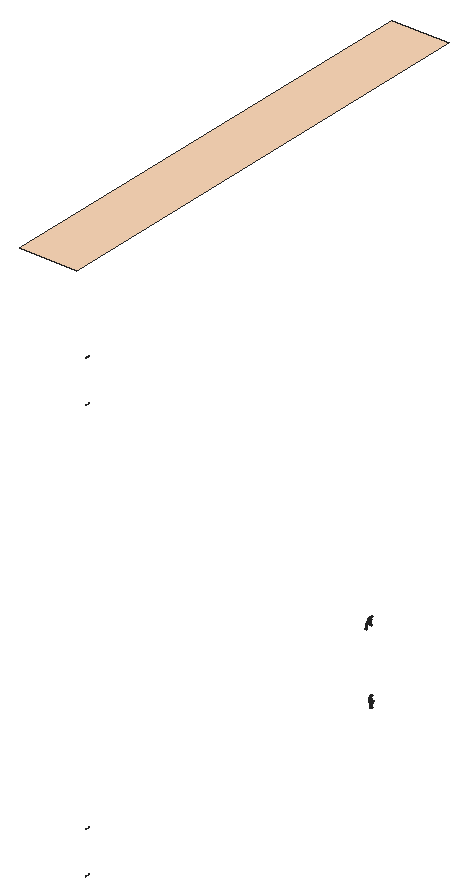
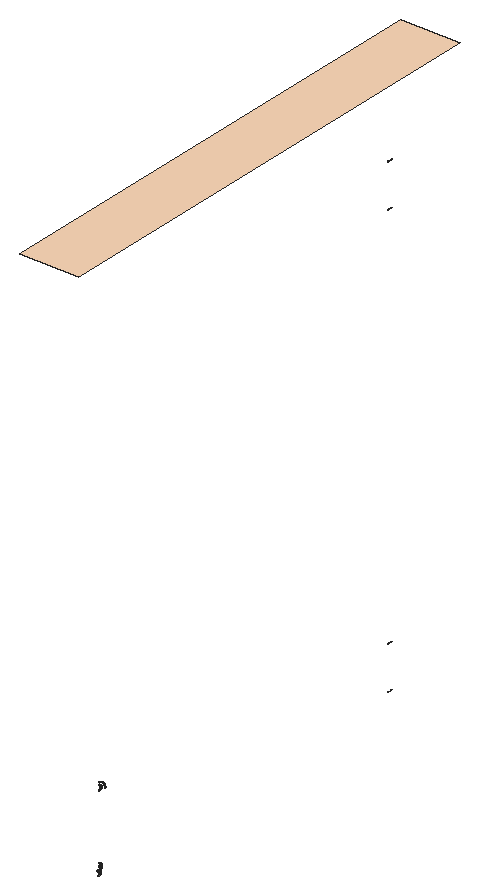
# SketchUp Ruby script. Lengths in inches.
U = 1.inch
M = Sketchup.active_model
def pt(a) = Geom::Point3d.new(a.map { |v| v * U })
def face(e, loops, mat)
  f = e.add_face(loops[0].map { |a| pt(a) })
  loops[1..].each { |l| e.add_face(l.map { |a| pt(a) }).erase! }
  f.material = f.back_material = mat if mat
  f
end
# faces: each face lists its corners as indices into pts; further lists are holes
def faces(e, pts, list, mat = nil) = list.each { |f| face(e, (f[0].is_a?(Array) ? f : [f]).map { |l| l.map { |i| pts[i] } }, mat) }
# xy, xz, yz: faces in a plane at the given z, y or x. An outline is a flat list of corners, or four numbers for a rectangle; further outlines are holes
def ring(l) = l.size == 4 ? [[l[0], l[1]], [l[2], l[1]], [l[2], l[3]], [l[0], l[3]]] : l.each_slice(2).to_a
def flat(e, list, mat, &to3) = list.each { |f| face(e, (f[0].is_a?(Array) ? f : [f]).map { |l| ring(l).map { |u, v| to3.(u, v) } }, mat) }
def xy(e, z, list, mat = nil) = flat(e, list, mat) { |x, y| [x, y, z] }
def xz(e, y, list, mat = nil) = flat(e, list, mat) { |x, z| [x, y, z] }
def yz(e, x, list, mat = nil) = flat(e, list, mat) { |y, z| [x, y, z] }
def lines(e, pts, list) = list.each { |a, b| e.add_line(pt(pts[a]), pt(pts[b])) }
# prism: a flat outline (further loops are holes) pulled along v
def prism(e, loops, v, mat = nil)
  f = face(e, loops, mat); d = Geom::Vector3d.new(v.map { |x| x * U })
  f.pushpull(f.normal.samedirection?(d) ? d.length : -d.length)
end
def box(e, o, s, mat = nil) = prism(e, [[o, [o[0] + s[0], o[1], o[2]], [o[0] + s[0], o[1] + s[1], o[2]], [o[0], o[1] + s[1], o[2]]]], [0, 0, s[2]], mat)
def at(x, y, z, deg = 0) = Geom::Transformation.translation(pt([x, y, z])) * Geom::Transformation.rotation(ORIGIN, Z_AXIS, deg.degrees)
def axes(o, x, y, z) = Geom::Transformation.new([*x, 0, *y, 0, *z, 0, *pt(o).to_a, 1])
def part(name) = M.definitions.add(name)
# library, detail: a bought-in or finely detailed component or shape, given as its bounding box
def library(name, o, s) = part(name).tap { |d| box(d.entities, o, s) }
def detail(e, o, s) = box(e.add_group.entities, o, s)
def put(e, d, t, mat = nil) = e.add_instance(d, t).tap { |i| i.material = mat if mat }
def group(e, t, mat = nil) = e.add_group.tap { |g| g.transformation = t; g.material = mat if mat }.entities
root = M.entities
M.materials.add("Material \#1").color = [140, 140, 140]
M.materials.add("[0027_PeachPuff]").color = [255, 218, 185]
xy(root,47.1053,[[362.6071,164.2401,362.6036,164.2537,362.604,164.275],[362.6071,164.2401,362.604,164.275,362.6071,164.2627],[362.6071,164.2401,362.6071,164.2627,362.6107,164.2537],[362.6036,164.2537,362.6005,164.293,362.6012,164.3103],[362.6036,164.2537,362.6012,164.3103,362.604,164.275],
  [362.6107,164.2537,362.6071,164.2627,362.6103,164.275],[362.6107,164.2537,362.6103,164.275,362.6137,164.293],[362.6103,164.275,362.6131,164.3103,362.6137,164.293],[362.6005,164.293,362.5982,164.3532,362.5991,164.3645],[362.6005,164.293,362.5991,164.3645,362.6012,164.3103],
  [362.6137,164.293,362.6131,164.3103,362.616,164.3532],[362.6131,164.3103,362.6152,164.3645,362.616,164.3532],[362.5982,164.3532,362.597,164.427,362.598,164.431],[362.5982,164.3532,362.598,164.431,362.5991,164.3645],[362.616,164.3532,362.6152,164.3645,362.6173,164.427],
  [362.6152,164.3645,362.6163,164.431,362.6173,164.427],[362.597,164.427,362.597,164.5056,362.598,164.5017],[362.597,164.427,362.598,164.5017,362.598,164.431],[362.6173,164.427,362.6163,164.431,362.6173,164.5056],[362.6163,164.431,362.6163,164.5017,362.6173,164.5056],
  [362.598,164.5017,362.597,164.5056,362.5991,164.5681],[362.6163,164.5017,362.6152,164.5681,362.616,164.5795],[362.6163,164.5017,362.616,164.5795,362.6173,164.5056],[362.597,164.5056,362.5982,164.5795,362.5991,164.5681],[362.5991,164.5681,362.5982,164.5795,362.6012,164.6223],
  [362.6152,164.5681,362.6131,164.6223,362.6137,164.6396],[362.6152,164.5681,362.6137,164.6396,362.616,164.5795],[362.5982,164.5795,362.6005,164.6396,362.6012,164.6223],[362.6012,164.6223,362.6005,164.6396,362.604,164.6577],[362.6131,164.6223,362.6103,164.6577,362.6107,164.6789],
  [362.6131,164.6223,362.6107,164.6789,362.6137,164.6396],[362.6005,164.6396,362.6036,164.6789,362.604,164.6577],[362.604,164.6577,362.6036,164.6789,362.6071,164.6699],[362.6103,164.6577,362.6071,164.6699,362.6071,164.6926],[362.6103,164.6577,362.6071,164.6926,362.6107,164.6789],
  [362.6071,164.6699,362.6036,164.6789,362.6071,164.6926]],"Material \#1")
xy(root,47.125,[[362.6071,164.2401,362.6071,164.2627,362.6036,164.2537],[362.6071,164.2401,362.6103,164.275,362.6071,164.2627],[362.6071,164.2401,362.6107,164.2537,362.6103,164.275],[362.6036,164.2537,362.604,164.275,362.6005,164.293],[362.6036,164.2537,362.6071,164.2627,362.604,164.275],
  [362.6107,164.2537,362.6131,164.3103,362.6103,164.275],[362.6107,164.2537,362.6137,164.293,362.6131,164.3103],[362.604,164.275,362.6012,164.3103,362.6005,164.293],[362.6005,164.293,362.6012,164.3103,362.5982,164.3532],[362.6137,164.293,362.6152,164.3645,362.6131,164.3103],
  [362.6137,164.293,362.616,164.3532,362.6152,164.3645],[362.6012,164.3103,362.5991,164.3645,362.5982,164.3532],[362.5982,164.3532,362.5991,164.3645,362.597,164.427],[362.616,164.3532,362.6163,164.431,362.6152,164.3645],[362.616,164.3532,362.6173,164.427,362.6163,164.431],
  [362.5991,164.3645,362.598,164.431,362.597,164.427],[362.597,164.427,362.598,164.431,362.597,164.5056],[362.6173,164.427,362.6163,164.5017,362.6163,164.431],[362.6173,164.427,362.6173,164.5056,362.6163,164.5017],[362.598,164.431,362.598,164.5017,362.597,164.5056],
  [362.598,164.5017,362.5982,164.5795,362.597,164.5056],[362.598,164.5017,362.5991,164.5681,362.5982,164.5795],[362.6163,164.5017,362.6173,164.5056,362.6152,164.5681],[362.6173,164.5056,362.616,164.5795,362.6152,164.5681],[362.5991,164.5681,362.6005,164.6396,362.5982,164.5795],
  [362.5991,164.5681,362.6012,164.6223,362.6005,164.6396],[362.6152,164.5681,362.616,164.5795,362.6131,164.6223],[362.616,164.5795,362.6137,164.6396,362.6131,164.6223],[362.6012,164.6223,362.6036,164.6789,362.6005,164.6396],[362.6012,164.6223,362.604,164.6577,362.6036,164.6789],
  [362.6131,164.6223,362.6137,164.6396,362.6103,164.6577],[362.6137,164.6396,362.6107,164.6789,362.6103,164.6577],[362.604,164.6577,362.6071,164.6926,362.6036,164.6789],[362.604,164.6577,362.6071,164.6699,362.6071,164.6926],[362.6103,164.6577,362.6107,164.6789,362.6071,164.6699],
  [362.6071,164.6699,362.6107,164.6789,362.6071,164.6926]],"Material \#1")
xy(root,51.5484,[[362.6071,164.2401,362.6036,164.2537,362.6071,164.2627],[362.6071,164.2401,362.6071,164.2627,362.6103,164.275],[362.6071,164.2401,362.6103,164.275,362.6107,164.2537],[362.6036,164.2537,362.6005,164.293,362.604,164.275],[362.6036,164.2537,362.604,164.275,362.6071,164.2627],
  [362.6107,164.2537,362.6103,164.275,362.6131,164.3103],[362.6107,164.2537,362.6131,164.3103,362.6137,164.293],[362.604,164.275,362.6005,164.293,362.6012,164.3103],[362.6005,164.293,362.5982,164.3532,362.6012,164.3103],[362.6137,164.293,362.6131,164.3103,362.6152,164.3645],
  [362.6137,164.293,362.6152,164.3645,362.616,164.3532],[362.6012,164.3103,362.5982,164.3532,362.5991,164.3645],[362.5982,164.3532,362.597,164.427,362.5991,164.3645],[362.616,164.3532,362.6152,164.3645,362.6163,164.431],[362.616,164.3532,362.6163,164.431,362.6173,164.427],
  [362.5991,164.3645,362.597,164.427,362.598,164.431],[362.597,164.427,362.597,164.5056,362.598,164.431],[362.6173,164.427,362.6163,164.431,362.6163,164.5017],[362.6173,164.427,362.6163,164.5017,362.6173,164.5056],[362.598,164.431,362.597,164.5056,362.598,164.5017],
  [362.598,164.5017,362.597,164.5056,362.5982,164.5794],[362.598,164.5017,362.5982,164.5794,362.5991,164.5681],[362.6163,164.5017,362.6152,164.5681,362.6173,164.5056],[362.6173,164.5056,362.6152,164.5681,362.616,164.5794],[362.5991,164.5681,362.5982,164.5794,362.6005,164.6396],
  [362.5991,164.5681,362.6005,164.6396,362.6012,164.6223],[362.6152,164.5681,362.6131,164.6223,362.616,164.5794],[362.616,164.5794,362.6131,164.6223,362.6137,164.6396],[362.6012,164.6223,362.6005,164.6396,362.6036,164.6789],[362.6012,164.6223,362.6036,164.6789,362.604,164.6577],
  [362.6131,164.6223,362.6103,164.6577,362.6137,164.6396],[362.6137,164.6396,362.6103,164.6577,362.6107,164.6789],[362.604,164.6577,362.6036,164.6789,362.6071,164.6926],[362.604,164.6577,362.6071,164.6926,362.6071,164.6699],[362.6103,164.6577,362.6071,164.6699,362.6107,164.6789],
  [362.6071,164.6699,362.6071,164.6926,362.6107,164.6789]],"Material \#1")
xy(root,51.5681,[[362.6071,164.2401,362.604,164.275,362.6036,164.2537],[362.6071,164.2401,362.6071,164.2627,362.604,164.275],[362.6071,164.2401,362.6107,164.2537,362.6071,164.2627],[362.6036,164.2537,362.6012,164.3103,362.6005,164.293],[362.6036,164.2537,362.604,164.275,362.6012,164.3103],
  [362.6107,164.2537,362.6103,164.275,362.6071,164.2627],[362.6107,164.2537,362.6137,164.293,362.6103,164.275],[362.6103,164.275,362.6137,164.293,362.6131,164.3103],[362.6005,164.293,362.5991,164.3645,362.5982,164.3532],[362.6005,164.293,362.6012,164.3103,362.5991,164.3645],
  [362.6137,164.293,362.616,164.3532,362.6131,164.3103],[362.6131,164.3103,362.616,164.3532,362.6152,164.3645],[362.5982,164.3532,362.598,164.431,362.597,164.427],[362.5982,164.3532,362.5991,164.3645,362.598,164.431],[362.616,164.3532,362.6173,164.427,362.6152,164.3645],
  [362.6152,164.3645,362.6173,164.427,362.6163,164.431],[362.597,164.427,362.598,164.431,362.598,164.5017],[362.597,164.427,362.598,164.5017,362.597,164.5056],[362.6173,164.427,362.6173,164.5056,362.6163,164.431],[362.6163,164.431,362.6173,164.5056,362.6163,164.5017],
  [362.598,164.5017,362.5991,164.5681,362.597,164.5056],[362.6163,164.5017,362.616,164.5794,362.6152,164.5681],[362.6163,164.5017,362.6173,164.5056,362.616,164.5794],[362.597,164.5056,362.5991,164.5681,362.5982,164.5794],[362.5991,164.5681,362.6012,164.6223,362.5982,164.5794],
  [362.6152,164.5681,362.6137,164.6396,362.6131,164.6223],[362.6152,164.5681,362.616,164.5794,362.6137,164.6396],[362.5982,164.5794,362.6012,164.6223,362.6005,164.6396],[362.6012,164.6223,362.604,164.6577,362.6005,164.6396],[362.6131,164.6223,362.6107,164.6789,362.6103,164.6577],
  [362.6131,164.6223,362.6137,164.6396,362.6107,164.6789],[362.6005,164.6396,362.604,164.6577,362.6036,164.6789],[362.604,164.6577,362.6071,164.6699,362.6036,164.6789],[362.6103,164.6577,362.6071,164.6926,362.6071,164.6699],[362.6103,164.6577,362.6107,164.6789,362.6071,164.6926],
  [362.6071,164.6699,362.6071,164.6926,362.6036,164.6789]],"Material \#1")
xy(root,91.4868,[[362.6071,164.2401,362.6036,164.2537,362.604,164.275],[362.6071,164.2401,362.604,164.275,362.6071,164.2627],[362.6071,164.2401,362.6071,164.2627,362.6107,164.2537],[362.6036,164.2537,362.6005,164.293,362.6012,164.3103],[362.6036,164.2537,362.6012,164.3103,362.604,164.275],
  [362.6107,164.2537,362.6071,164.2627,362.6103,164.275],[362.6107,164.2537,362.6103,164.275,362.6137,164.293],[362.6103,164.275,362.6131,164.3103,362.6137,164.293],[362.6005,164.293,362.5982,164.3532,362.5991,164.3645],[362.6005,164.293,362.5991,164.3645,362.6012,164.3103],
  [362.6137,164.293,362.6131,164.3103,362.616,164.3532],[362.6131,164.3103,362.6152,164.3645,362.616,164.3532],[362.5982,164.3532,362.597,164.427,362.598,164.431],[362.5982,164.3532,362.598,164.431,362.5991,164.3645],[362.616,164.3532,362.6152,164.3645,362.6173,164.427],
  [362.6152,164.3645,362.6163,164.431,362.6173,164.427],[362.597,164.427,362.597,164.5056,362.598,164.5017],[362.597,164.427,362.598,164.5017,362.598,164.431],[362.6173,164.427,362.6163,164.431,362.6173,164.5056],[362.6163,164.431,362.6163,164.5017,362.6173,164.5056],
  [362.598,164.5017,362.597,164.5056,362.5991,164.5681],[362.6163,164.5017,362.6152,164.5681,362.616,164.5794],[362.6163,164.5017,362.616,164.5794,362.6173,164.5056],[362.597,164.5056,362.5982,164.5794,362.5991,164.5681],[362.5991,164.5681,362.5982,164.5794,362.6012,164.6223],
  [362.6152,164.5681,362.6131,164.6223,362.6137,164.6396],[362.6152,164.5681,362.6137,164.6396,362.616,164.5794],[362.5982,164.5794,362.6005,164.6396,362.6012,164.6223],[362.6012,164.6223,362.6005,164.6396,362.604,164.6577],[362.6131,164.6223,362.6103,164.6577,362.6107,164.6789],
  [362.6131,164.6223,362.6107,164.6789,362.6137,164.6396],[362.6005,164.6396,362.6036,164.6789,362.604,164.6577],[362.604,164.6577,362.6036,164.6789,362.6071,164.6699],[362.6103,164.6577,362.6071,164.6699,362.6071,164.6926],[362.6103,164.6577,362.6071,164.6926,362.6107,164.6789],
  [362.6071,164.6699,362.6036,164.6789,362.6071,164.6926]],"Material \#1")
xy(root,91.5065,[[362.6071,164.2401,362.6071,164.2627,362.6036,164.2537],[362.6071,164.2401,362.6103,164.275,362.6071,164.2627],[362.6071,164.2401,362.6107,164.2537,362.6103,164.275],[362.6036,164.2537,362.604,164.275,362.6005,164.293],[362.6036,164.2537,362.6071,164.2627,362.604,164.275],
  [362.6107,164.2537,362.6131,164.3103,362.6103,164.275],[362.6107,164.2537,362.6137,164.293,362.6131,164.3103],[362.604,164.275,362.6012,164.3103,362.6005,164.293],[362.6005,164.293,362.6012,164.3103,362.5982,164.3532],[362.6137,164.293,362.6152,164.3645,362.6131,164.3103],
  [362.6137,164.293,362.616,164.3532,362.6152,164.3645],[362.6012,164.3103,362.5991,164.3645,362.5982,164.3532],[362.5982,164.3532,362.5991,164.3645,362.597,164.427],[362.616,164.3532,362.6163,164.431,362.6152,164.3645],[362.616,164.3532,362.6173,164.427,362.6163,164.431],
  [362.5991,164.3645,362.598,164.431,362.597,164.427],[362.597,164.427,362.598,164.431,362.597,164.5056],[362.6173,164.427,362.6163,164.5017,362.6163,164.431],[362.6173,164.427,362.6173,164.5056,362.6163,164.5017],[362.598,164.431,362.598,164.5017,362.597,164.5056],
  [362.598,164.5017,362.5982,164.5794,362.597,164.5056],[362.598,164.5017,362.5991,164.5681,362.5982,164.5794],[362.6163,164.5017,362.6173,164.5056,362.6152,164.5681],[362.6173,164.5056,362.616,164.5794,362.6152,164.5681],[362.5991,164.5681,362.6005,164.6396,362.5982,164.5794],
  [362.5991,164.5681,362.6012,164.6223,362.6005,164.6396],[362.6152,164.5681,362.616,164.5794,362.6131,164.6223],[362.616,164.5794,362.6137,164.6396,362.6131,164.6223],[362.6012,164.6223,362.6036,164.6789,362.6005,164.6396],[362.6012,164.6223,362.604,164.6577,362.6036,164.6789],
  [362.6131,164.6223,362.6137,164.6396,362.6103,164.6577],[362.6137,164.6396,362.6107,164.6789,362.6103,164.6577],[362.604,164.6577,362.6071,164.6926,362.6036,164.6789],[362.604,164.6577,362.6071,164.6699,362.6071,164.6926],[362.6103,164.6577,362.6107,164.6789,362.6071,164.6699],
  [362.6071,164.6699,362.6107,164.6789,362.6071,164.6926]],"Material \#1")
xy(root,95.9299,[[362.6071,164.2401,362.6036,164.2537,362.6071,164.2627],[362.6071,164.2401,362.6071,164.2627,362.6103,164.275],[362.6071,164.2401,362.6103,164.275,362.6107,164.2537],[362.6036,164.2537,362.6005,164.293,362.604,164.275],[362.6036,164.2537,362.604,164.275,362.6071,164.2627],
  [362.6107,164.2537,362.6103,164.275,362.6131,164.3103],[362.6107,164.2537,362.6131,164.3103,362.6137,164.293],[362.604,164.275,362.6005,164.293,362.6012,164.3103],[362.6005,164.293,362.5982,164.3532,362.6012,164.3103],[362.6137,164.293,362.6131,164.3103,362.6152,164.3645],
  [362.6137,164.293,362.6152,164.3645,362.616,164.3532],[362.6012,164.3103,362.5982,164.3532,362.5991,164.3645],[362.5982,164.3532,362.597,164.427,362.5991,164.3645],[362.616,164.3532,362.6152,164.3645,362.6163,164.431],[362.616,164.3532,362.6163,164.431,362.6173,164.427],
  [362.5991,164.3645,362.597,164.427,362.598,164.431],[362.597,164.427,362.597,164.5056,362.598,164.431],[362.6173,164.427,362.6163,164.431,362.6163,164.5017],[362.6173,164.427,362.6163,164.5017,362.6173,164.5056],[362.598,164.431,362.597,164.5056,362.598,164.5017],
  [362.598,164.5017,362.597,164.5056,362.5982,164.5794],[362.598,164.5017,362.5982,164.5794,362.5991,164.5681],[362.6163,164.5017,362.6152,164.5681,362.6173,164.5056],[362.6173,164.5056,362.6152,164.5681,362.616,164.5794],[362.5991,164.5681,362.5982,164.5794,362.6005,164.6396],
  [362.5991,164.5681,362.6005,164.6396,362.6012,164.6223],[362.6152,164.5681,362.6131,164.6223,362.616,164.5794],[362.616,164.5794,362.6131,164.6223,362.6137,164.6396],[362.6012,164.6223,362.6005,164.6396,362.6036,164.6789],[362.6012,164.6223,362.6036,164.6789,362.604,164.6577],
  [362.6131,164.6223,362.6103,164.6577,362.6137,164.6396],[362.6137,164.6396,362.6103,164.6577,362.6107,164.6789],[362.604,164.6577,362.6036,164.6789,362.6071,164.6926],[362.604,164.6577,362.6071,164.6926,362.6071,164.6699],[362.6103,164.6577,362.6071,164.6699,362.6107,164.6789],
  [362.6071,164.6699,362.6071,164.6926,362.6107,164.6789]],"Material \#1")
xy(root,95.9497,[[362.6071,164.2401,362.604,164.275,362.6036,164.2537],[362.6071,164.2401,362.6071,164.2627,362.604,164.275],[362.6071,164.2401,362.6107,164.2537,362.6071,164.2627],[362.6036,164.2537,362.6012,164.3103,362.6005,164.293],[362.6036,164.2537,362.604,164.275,362.6012,164.3103],
  [362.6107,164.2537,362.6103,164.275,362.6071,164.2627],[362.6107,164.2537,362.6137,164.293,362.6103,164.275],[362.6103,164.275,362.6137,164.293,362.6131,164.3103],[362.6005,164.293,362.5991,164.3645,362.5982,164.3532],[362.6005,164.293,362.6012,164.3103,362.5991,164.3645],
  [362.6137,164.293,362.616,164.3532,362.6131,164.3103],[362.6131,164.3103,362.616,164.3532,362.6152,164.3645],[362.5982,164.3532,362.598,164.431,362.597,164.427],[362.5982,164.3532,362.5991,164.3645,362.598,164.431],[362.616,164.3532,362.6173,164.427,362.6152,164.3645],
  [362.6152,164.3645,362.6173,164.427,362.6163,164.431],[362.597,164.427,362.598,164.431,362.598,164.5017],[362.597,164.427,362.598,164.5017,362.597,164.5056],[362.6173,164.427,362.6173,164.5056,362.6163,164.431],[362.6163,164.431,362.6173,164.5056,362.6163,164.5017],
  [362.598,164.5017,362.5991,164.5681,362.597,164.5056],[362.6163,164.5017,362.616,164.5794,362.6152,164.5681],[362.6163,164.5017,362.6173,164.5056,362.616,164.5794],[362.597,164.5056,362.5991,164.5681,362.5982,164.5794],[362.5991,164.5681,362.6012,164.6223,362.5982,164.5794],
  [362.6152,164.5681,362.6137,164.6396,362.6131,164.6223],[362.6152,164.5681,362.616,164.5794,362.6137,164.6396],[362.5982,164.5794,362.6012,164.6223,362.6005,164.6396],[362.6012,164.6223,362.604,164.6577,362.6005,164.6396],[362.6131,164.6223,362.6107,164.6789,362.6103,164.6577],
  [362.6131,164.6223,362.6137,164.6396,362.6107,164.6789],[362.6005,164.6396,362.604,164.6577,362.6036,164.6789],[362.604,164.6577,362.6071,164.6699,362.6036,164.6789],[362.6103,164.6577,362.6071,164.6926,362.6071,164.6699],[362.6103,164.6577,362.6107,164.6789,362.6071,164.6926],
  [362.6071,164.6699,362.6071,164.6926,362.6036,164.6789]],"Material \#1")
xy(root,106.4375,[[358.5625,160.62,364.5625,209.4903]],"[0027_PeachPuff]")
xz(root,201.7613,[[362.5633,47.3132,362.5825,47.3132,362.5825,47.3412],[362.5633,47.3132,362.5825,47.3412,362.5633,47.3412],[362.6688,47.3132,362.688,47.3132,362.6688,47.3412],[362.688,47.3132,362.688,47.3412,362.6688,47.3412]],"Material \#1")
yz(root,362.5639,[[201.6636,46.5567,201.7978,47.0437,201.6258,46.6739],[201.6258,46.6739,201.628,47.1087,201.6258,47.0323],[201.6258,46.6739,201.6784,47.0737,201.628,47.1087],[201.6258,46.6739,201.7356,47.0515,201.6784,47.0737],[201.6258,46.6739,201.7978,47.0437,201.7356,47.0515],
  [201.6258,47.0323,201.624,47.048,201.6254,47.0405],[201.6258,47.0323,201.628,47.1087,201.624,47.048],[201.624,47.048,201.586,47.1545,201.6188,47.0615],[201.624,47.048,201.628,47.1087,201.586,47.1545],[201.624,47.048,201.6188,47.0615,201.6219,47.055],
  [201.6188,47.0615,201.4929,47.2953,201.615,47.0675],[201.6188,47.0615,201.5539,47.2095,201.4929,47.2953],[201.6188,47.0615,201.586,47.1545,201.5539,47.2095],[201.615,47.0675,201.4929,47.2953,201.6103,47.0733],[201.6103,47.0733,201.4929,47.2953,201.5523,47.1402],
  [201.6103,47.0733,201.5523,47.1402,201.6049,47.0789],[201.6049,47.0789,201.5523,47.1402,201.5771,47.108],[201.5523,47.1402,201.4929,47.2953,201.5138,47.213],[201.5523,47.1402,201.5138,47.213,201.5311,47.1753],[201.5539,47.2095,201.5334,47.2717,201.4929,47.2953],
  [201.5138,47.213,201.4929,47.2953,201.5009,47.2531],[201.5334,47.2717,201.5263,47.3395,201.4929,47.2953],[201.4929,47.2953,201.4982,47.4164,201.4901,47.3395],[201.4929,47.2953,201.5263,47.3395,201.5334,47.4073],[201.4929,47.2953,201.5334,47.4073,201.5539,47.4696],
  [201.4929,47.2953,201.5539,47.4696,201.5577,47.5492],[201.4929,47.2953,201.5577,47.5492,201.4982,47.4164],[201.4982,47.4164,201.5577,47.5492,201.5214,47.4869],[201.5539,47.4696,201.586,47.5245,201.5577,47.5492],[201.586,47.5245,201.628,47.5704,201.5577,47.5492],
  [201.5577,47.5492,201.628,47.5704,201.6784,47.6053],[201.5577,47.5492,201.6625,47.6407,201.6054,47.6011],[201.5577,47.5492,201.6784,47.6053,201.7978,47.6749],[201.5577,47.5492,201.7978,47.6749,201.6625,47.6407],[201.6784,47.6053,201.7356,47.6276,201.7978,47.6749],
  [201.7356,47.6276,201.7978,47.6354,201.7978,47.6749],[201.6625,47.6407,201.7978,47.6749,201.7273,47.666]],"Material \#1")
yz(root,362.566,[[201.0195,54.2371,201.0325,54.3958,201.0059,54.2378],[201.0059,54.2378,201.0325,54.3958,201.0191,54.3984],[201.7507,54.3066,201.7109,54.3338,201.7061,54.3199],[201.7507,54.3066,201.7532,54.3212,201.7109,54.3338],[201.7061,54.3199,201.6719,54.354,201.665,54.3412],
  [201.7061,54.3199,201.7109,54.3338,201.6719,54.354],[201.665,54.3412,201.6372,54.3808,201.6284,54.3695],[201.665,54.3412,201.6719,54.354,201.6372,54.3808],[201.6284,54.3695,201.6072,54.4135,201.5967,54.4039],[201.6284,54.3695,201.6372,54.3808,201.6072,54.4135],
  [201.0325,54.3958,201.0686,54.539,201.0191,54.3984],[201.0191,54.3984,201.0686,54.539,201.0559,54.5441],[201.5967,54.4039,201.5826,54.4514,201.5708,54.4439],[201.5967,54.4039,201.6072,54.4135,201.5826,54.4514],[201.5708,54.4439,201.5641,54.4938,201.5513,54.4886],
  [201.5708,54.4439,201.5826,54.4514,201.5641,54.4938],[201.5513,54.4886,201.5524,54.5399,201.539,54.5373],[201.5513,54.4886,201.5641,54.4938,201.5524,54.5399],[201.539,54.5373,201.5484,54.5885,201.5348,54.5885],[201.539,54.5373,201.5524,54.5399,201.5484,54.5885],
  [201.0686,54.539,201.1262,54.6709,201.0559,54.5441],[201.0559,54.5441,201.1262,54.6709,201.1144,54.6784],[201.5348,54.5885,201.5484,54.5885,201.5524,54.6371],[201.5348,54.5885,201.5524,54.6371,201.539,54.6398],[201.5524,54.6371,201.5641,54.6832,201.539,54.6398],
  [201.539,54.6398,201.5641,54.6832,201.5513,54.6884],[201.1262,54.6709,201.203,54.7892,201.1144,54.6784],[201.1144,54.6784,201.203,54.7892,201.1926,54.7988],[201.5641,54.6832,201.5826,54.7257,201.5513,54.6884],[201.5513,54.6884,201.5826,54.7257,201.5708,54.7332],
  [201.5826,54.7257,201.6072,54.7636,201.5708,54.7332],[201.5708,54.7332,201.6072,54.7636,201.5967,54.7731],[201.6072,54.7636,201.6372,54.7962,201.5967,54.7731],[201.5967,54.7731,201.6372,54.7962,201.6284,54.8076],[201.203,54.7892,201.2968,54.8915,201.1926,54.7988],
  [201.6372,54.7962,201.6719,54.823,201.6284,54.8076],[201.1926,54.7988,201.2968,54.8915,201.288,54.9029],[201.6284,54.8076,201.6719,54.823,201.665,54.8358],[201.6719,54.823,201.7109,54.8432,201.665,54.8358],[201.665,54.8358,201.7109,54.8432,201.7061,54.8571],
  [201.7109,54.8432,201.7532,54.8559,201.7061,54.8571],[201.7532,54.8559,201.7507,54.8705,201.7061,54.8571],[201.2968,54.8915,201.4054,54.9752,201.288,54.9029],[201.288,54.9029,201.4054,54.9752,201.3986,54.988],[201.4054,54.9752,201.5265,55.0379,201.3986,54.988],
  [201.3986,54.988,201.5265,55.0379,201.5217,55.0518],[201.5265,55.0379,201.6578,55.0773,201.5217,55.0518],[201.5217,55.0518,201.6578,55.0773,201.6554,55.0919],[201.6578,55.0773,201.7978,55.0909,201.6554,55.0919],[201.7978,55.0909,201.7978,55.1058,201.6554,55.0919]],"Material \#1")
yz(root,362.5845,[[201.7978,46.4864,201.7584,46.4914,201.7222,46.5055],[201.7222,46.5055,201.6304,46.6309,201.8734,46.5055],[201.7222,46.5055,201.6636,46.5567,201.6304,46.6309],[201.7222,46.5055,201.6903,46.5276,201.6636,46.5567],[201.6636,46.5567,201.6433,46.5915,201.6304,46.6309],
  [201.6304,46.6309,201.6258,46.6739,201.9763,47.0609],[201.6258,46.6739,201.6258,47.0323,201.7356,47.0515],[201.6258,46.6739,201.7356,47.0515,201.7978,47.0436],[201.6258,46.6739,201.7978,47.0436,201.86,47.0515],[201.6258,47.0323,201.624,47.048,201.7356,47.0515],
  [201.6258,47.0323,201.6254,47.0405,201.624,47.048],[201.624,47.048,201.6188,47.0615,201.7356,47.0515],[201.624,47.048,201.6219,47.055,201.6188,47.0615],[201.7356,47.0515,201.6188,47.0615,201.6784,47.0737],[201.6188,47.0615,201.4929,47.2953,201.586,47.1545],
  [201.6188,47.0615,201.615,47.0675,201.4929,47.2953],[201.6188,47.0615,201.586,47.1545,201.628,47.1087],[201.6188,47.0615,201.628,47.1087,201.6784,47.0737],[201.615,47.0675,201.6103,47.0733,201.4929,47.2953],[201.6103,47.0733,201.5524,47.1402,201.4929,47.2953],
  [201.6103,47.0733,201.6049,47.0789,201.5524,47.1402],[201.6049,47.0789,201.5771,47.108,201.5524,47.1402],[201.5524,47.1402,201.5138,47.213,201.4929,47.2953],[201.5524,47.1402,201.5311,47.1753,201.5138,47.213],[201.586,47.1545,201.4929,47.2953,201.5539,47.2095],
  [201.5539,47.2095,201.4929,47.2953,201.5334,47.2717],[201.5138,47.213,201.5009,47.2531,201.4929,47.2953],[201.5334,47.2717,201.4929,47.2953,201.5263,47.3395],[201.4929,47.2953,201.4901,47.3395,201.4982,47.4164],[201.4929,47.2953,201.4982,47.4164,201.5577,47.5492],
  [201.4929,47.2953,201.5334,47.4073,201.5263,47.3395],[201.4929,47.2953,201.5577,47.5492,201.5334,47.4073],[201.5334,47.4073,201.5577,47.5492,201.5539,47.4696],[201.4982,47.4164,201.5214,47.4869,201.5577,47.5492],[201.5539,47.4696,201.5577,47.5492,201.586,47.5245],
  [201.586,47.5245,201.5577,47.5492,201.628,47.5704],[201.5577,47.5492,201.6054,47.6011,201.6625,47.6407],[201.5577,47.5492,201.6625,47.6407,201.7978,47.6749],[201.5577,47.5492,201.6784,47.6053,201.628,47.5704],[201.5577,47.5492,201.7978,47.6749,201.6784,47.6053],
  [201.6784,47.6053,201.7978,47.6749,201.7356,47.6276],[201.6625,47.6407,201.7273,47.666,201.7978,47.6749]],"Material \#1")
yz(root,362.6668,[[201.7978,46.4864,201.7222,46.5055,201.7584,46.4914],[201.7222,46.5055,201.6304,46.6309,201.6636,46.5567],[201.7222,46.5055,201.8734,46.5055,201.6304,46.6309],[201.7222,46.5055,201.6636,46.5567,201.6903,46.5276],[201.6636,46.5567,201.6304,46.6309,201.6433,46.5915],
  [201.6304,46.6309,201.9763,47.0609,201.6258,46.6739],[201.6258,46.6739,201.7356,47.0515,201.6258,47.0323],[201.6258,46.6739,201.7978,47.0436,201.7356,47.0515],[201.6258,46.6739,201.86,47.0515,201.7978,47.0436],[201.6258,47.0323,201.624,47.048,201.6254,47.0405],
  [201.6258,47.0323,201.7356,47.0515,201.624,47.048],[201.624,47.048,201.6188,47.0615,201.6219,47.055],[201.624,47.048,201.7356,47.0515,201.6188,47.0615],[201.7356,47.0515,201.6784,47.0737,201.6188,47.0615],[201.6188,47.0615,201.4929,47.2953,201.615,47.0675],
  [201.6188,47.0615,201.586,47.1545,201.4929,47.2953],[201.6188,47.0615,201.628,47.1087,201.586,47.1545],[201.6188,47.0615,201.6784,47.0737,201.628,47.1087],[201.615,47.0675,201.4929,47.2953,201.6103,47.0733],[201.6103,47.0733,201.4929,47.2953,201.5524,47.1402],
  [201.6103,47.0733,201.5524,47.1402,201.6049,47.0789],[201.6049,47.0789,201.5524,47.1402,201.5771,47.108],[201.5524,47.1402,201.4929,47.2953,201.5138,47.213],[201.5524,47.1402,201.5138,47.213,201.5311,47.1753],[201.586,47.1545,201.5539,47.2095,201.4929,47.2953],
  [201.5539,47.2095,201.5334,47.2717,201.4929,47.2953],[201.5138,47.213,201.4929,47.2953,201.5009,47.2531],[201.5334,47.2717,201.5263,47.3395,201.4929,47.2953],[201.4929,47.2953,201.4982,47.4164,201.4901,47.3395],[201.4929,47.2953,201.5263,47.3395,201.5334,47.4073],
  [201.4929,47.2953,201.5334,47.4073,201.5577,47.5492],[201.4929,47.2953,201.5577,47.5492,201.4982,47.4164],[201.5334,47.4073,201.5539,47.4696,201.5577,47.5492],[201.4982,47.4164,201.5577,47.5492,201.5214,47.4869],[201.5539,47.4696,201.586,47.5245,201.5577,47.5492],
  [201.586,47.5245,201.628,47.5704,201.5577,47.5492],[201.5577,47.5492,201.628,47.5704,201.6784,47.6053],[201.5577,47.5492,201.6625,47.6407,201.6054,47.6011],[201.5577,47.5492,201.6784,47.6053,201.7978,47.6749],[201.5577,47.5492,201.7978,47.6749,201.6625,47.6407],
  [201.6784,47.6053,201.7356,47.6276,201.7978,47.6749],[201.6625,47.6407,201.7978,47.6749,201.7273,47.666]],"Material \#1")
yz(root,362.6853,[[201.0195,54.2371,201.0059,54.2378,201.0325,54.3958],[201.0059,54.2378,201.0191,54.3984,201.0325,54.3958],[201.7507,54.3066,201.7061,54.3199,201.7109,54.3338],[201.7507,54.3066,201.7109,54.3338,201.7532,54.3212],[201.7061,54.3199,201.665,54.3412,201.6719,54.354],
  [201.7061,54.3199,201.6719,54.354,201.7109,54.3338],[201.665,54.3412,201.6284,54.3695,201.6372,54.3808],[201.665,54.3412,201.6372,54.3808,201.6719,54.354],[201.6284,54.3695,201.5967,54.4039,201.6072,54.4135],[201.6284,54.3695,201.6072,54.4135,201.6372,54.3808],
  [201.0325,54.3958,201.0191,54.3984,201.0686,54.539],[201.0191,54.3984,201.0559,54.5441,201.0686,54.539],[201.5967,54.4039,201.5708,54.4439,201.5826,54.4514],[201.5967,54.4039,201.5826,54.4514,201.6072,54.4135],[201.5708,54.4439,201.5513,54.4886,201.5641,54.4938],
  [201.5708,54.4439,201.5641,54.4938,201.5826,54.4514],[201.5513,54.4886,201.539,54.5373,201.5524,54.5399],[201.5513,54.4886,201.5524,54.5399,201.5641,54.4938],[201.539,54.5373,201.5348,54.5885,201.5484,54.5885],[201.539,54.5373,201.5484,54.5885,201.5524,54.5399],
  [201.0686,54.539,201.0559,54.5441,201.1262,54.6709],[201.0559,54.5441,201.1144,54.6784,201.1262,54.6709],[201.5348,54.5885,201.539,54.6398,201.5524,54.6371],[201.5348,54.5885,201.5524,54.6371,201.5484,54.5885],[201.5524,54.6371,201.539,54.6398,201.5641,54.6832],
  [201.539,54.6398,201.5513,54.6884,201.5641,54.6832],[201.1262,54.6709,201.1144,54.6784,201.203,54.7892],[201.1144,54.6784,201.1926,54.7988,201.203,54.7892],[201.5641,54.6832,201.5513,54.6884,201.5826,54.7257],[201.5513,54.6884,201.5708,54.7332,201.5826,54.7257],
  [201.5826,54.7257,201.5708,54.7332,201.6072,54.7636],[201.5708,54.7332,201.5967,54.7731,201.6072,54.7636],[201.6072,54.7636,201.5967,54.7731,201.6372,54.7962],[201.5967,54.7731,201.6284,54.8076,201.6372,54.7962],[201.203,54.7892,201.1926,54.7988,201.2968,54.8915],
  [201.6372,54.7962,201.6284,54.8076,201.6719,54.823],[201.1926,54.7988,201.288,54.9029,201.2968,54.8915],[201.6284,54.8076,201.665,54.8358,201.6719,54.823],[201.6719,54.823,201.665,54.8358,201.7109,54.8432],[201.665,54.8358,201.7061,54.8571,201.7109,54.8432],
  [201.7109,54.8432,201.7061,54.8571,201.7532,54.8559],[201.7532,54.8559,201.7061,54.8571,201.7507,54.8705],[201.2968,54.8915,201.288,54.9029,201.4054,54.9752],[201.288,54.9029,201.3986,54.988,201.4054,54.9752],[201.4054,54.9752,201.3986,54.988,201.5265,55.0379],
  [201.3986,54.988,201.5217,55.0518,201.5265,55.0379],[201.5265,55.0379,201.5217,55.0518,201.6578,55.0773],[201.5217,55.0518,201.6554,55.0919,201.6578,55.0773],[201.6578,55.0773,201.6554,55.0919,201.7978,55.0909],[201.7978,55.0909,201.6554,55.0919,201.7978,55.1058]],"Material \#1")
yz(root,362.6874,[[201.7978,46.4864,201.7222,46.5055,201.6636,46.5567],[201.7978,46.4864,201.7584,46.4914,201.7222,46.5055],[201.7222,46.5055,201.6903,46.5276,201.6636,46.5567],[201.6636,46.5567,201.6258,46.6739,201.7978,47.0436],[201.6636,46.5567,201.6304,46.6309,201.6258,46.6739],
  [201.6636,46.5567,201.6433,46.5915,201.6304,46.6309],[201.6258,46.6739,201.6258,47.0323,201.628,47.1087],[201.6258,46.6739,201.628,47.1087,201.6784,47.0737],[201.6258,46.6739,201.6784,47.0737,201.7356,47.0515],[201.6258,46.6739,201.7356,47.0515,201.7978,47.0436],
  [201.6258,47.0323,201.624,47.048,201.628,47.1087],[201.6258,47.0323,201.6254,47.0405,201.624,47.048],[201.624,47.048,201.586,47.1545,201.628,47.1087],[201.624,47.048,201.6188,47.0615,201.586,47.1545],[201.624,47.048,201.6219,47.055,201.6188,47.0615],
  [201.6188,47.0615,201.4929,47.2953,201.5539,47.2095],[201.6188,47.0615,201.615,47.0675,201.4929,47.2953],[201.6188,47.0615,201.5539,47.2095,201.586,47.1545],[201.615,47.0675,201.6103,47.0733,201.4929,47.2953],[201.6103,47.0733,201.5523,47.1402,201.4929,47.2953],
  [201.6103,47.0733,201.6049,47.0789,201.5523,47.1402],[201.6049,47.0789,201.5771,47.108,201.5523,47.1402],[201.5523,47.1402,201.5138,47.213,201.4929,47.2953],[201.5523,47.1402,201.5311,47.1753,201.5138,47.213],[201.5539,47.2095,201.4929,47.2953,201.5334,47.2717],
  [201.5138,47.213,201.5009,47.2531,201.4929,47.2953],[201.5334,47.2717,201.4929,47.2953,201.5263,47.3395],[201.4929,47.2953,201.4901,47.3395,201.4982,47.4164],[201.4929,47.2953,201.4982,47.4164,201.5577,47.5492],[201.4929,47.2953,201.5334,47.4073,201.5263,47.3395],
  [201.4929,47.2953,201.5539,47.4696,201.5334,47.4073],[201.4929,47.2953,201.5577,47.5492,201.5539,47.4696],[201.4982,47.4164,201.5214,47.4869,201.5577,47.5492],[201.5539,47.4696,201.5577,47.5492,201.586,47.5245],[201.586,47.5245,201.5577,47.5492,201.628,47.5704],
  [201.5577,47.5492,201.6054,47.6011,201.6625,47.6407],[201.5577,47.5492,201.6625,47.6407,201.7978,47.6749],[201.5577,47.5492,201.6784,47.6053,201.628,47.5704],[201.5577,47.5492,201.7978,47.6749,201.6784,47.6053],[201.6784,47.6053,201.7978,47.6749,201.7356,47.6276],
  [201.6625,47.6407,201.7273,47.666,201.7978,47.6749]],"Material \#1")
p = [[362.5825,201.7613,47.3132],[362.5633,201.7613,47.3132],[362.5633,201.7713,47.2853],[362.5633,201.7613,47.3412],[362.5825,201.7613,47.3412],[362.5825,201.7713,47.3691],
  [362.6688,201.7713,47.3691],[362.6688,201.7613,47.3412],[362.688,201.7613,47.3412]]
faces(root,p,[[0,1,2],[3,4,5],[6,7,8]],"Material \#1")
